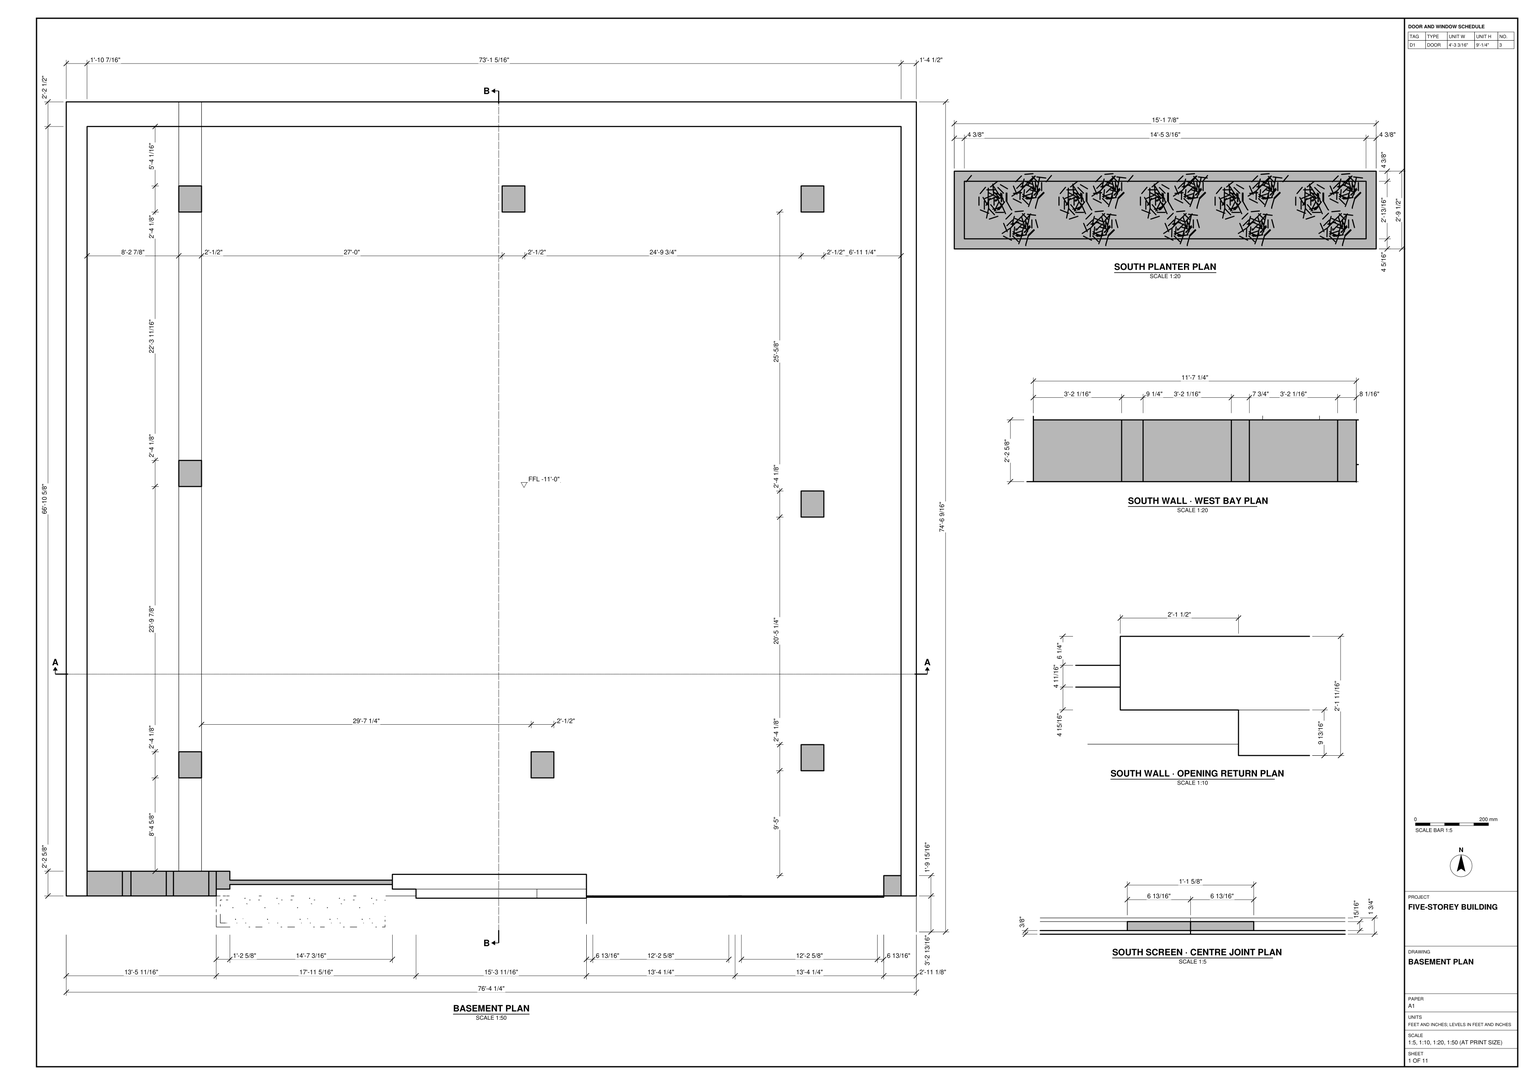
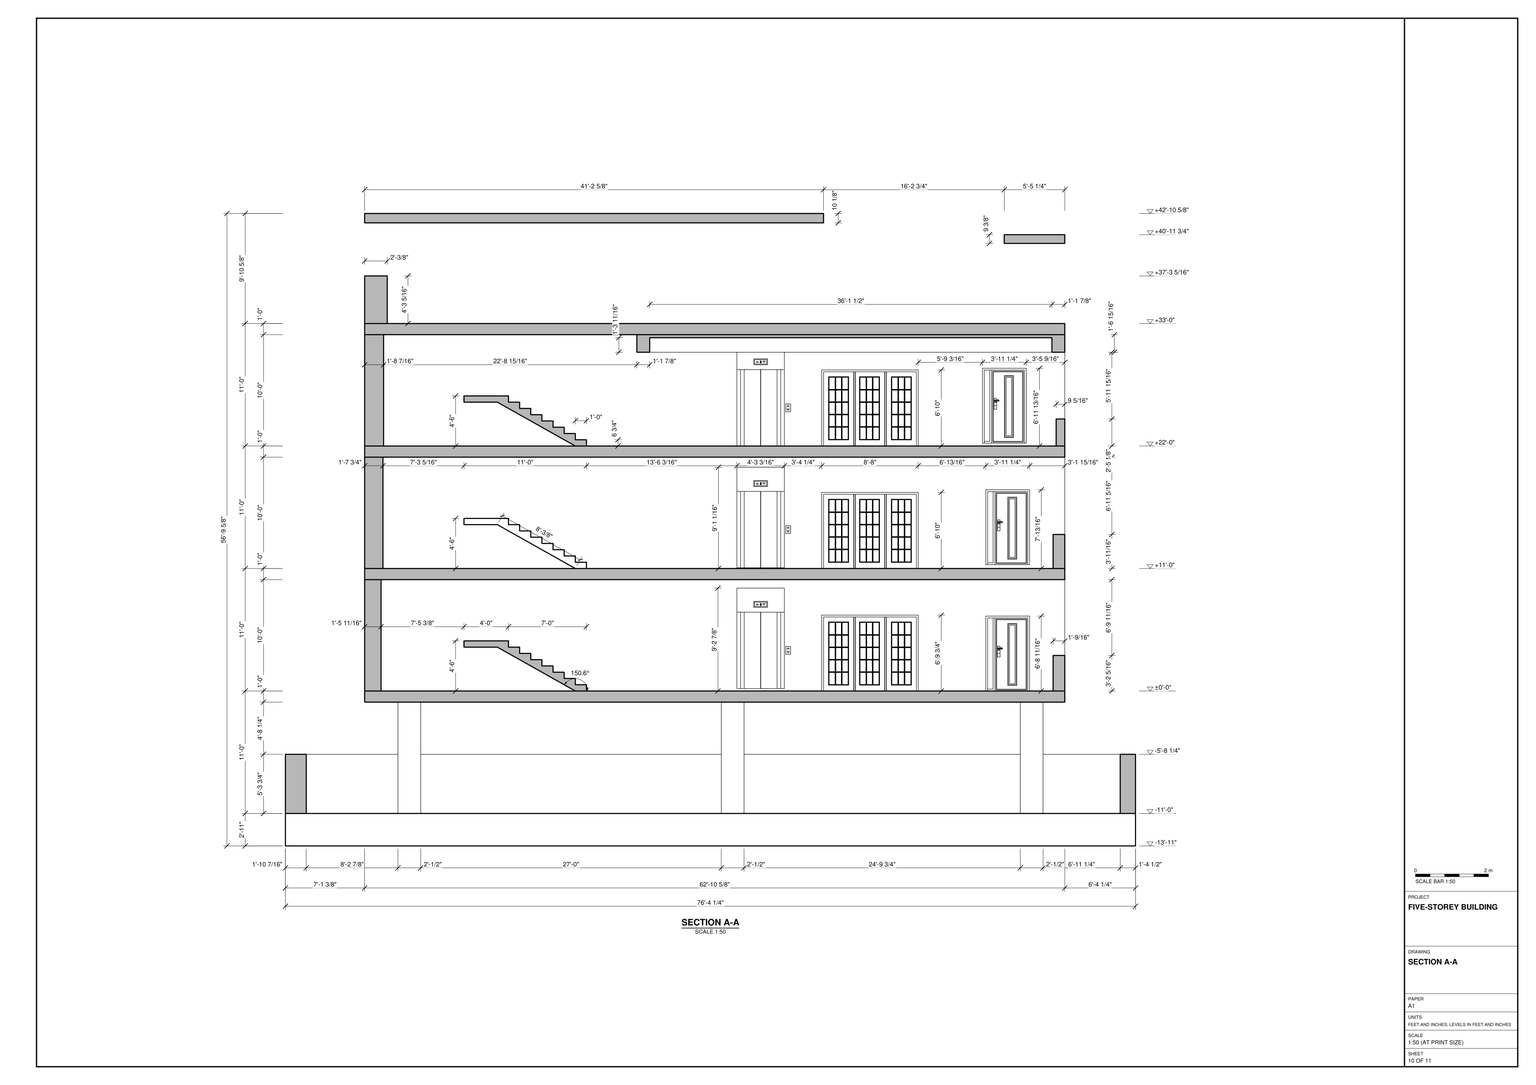
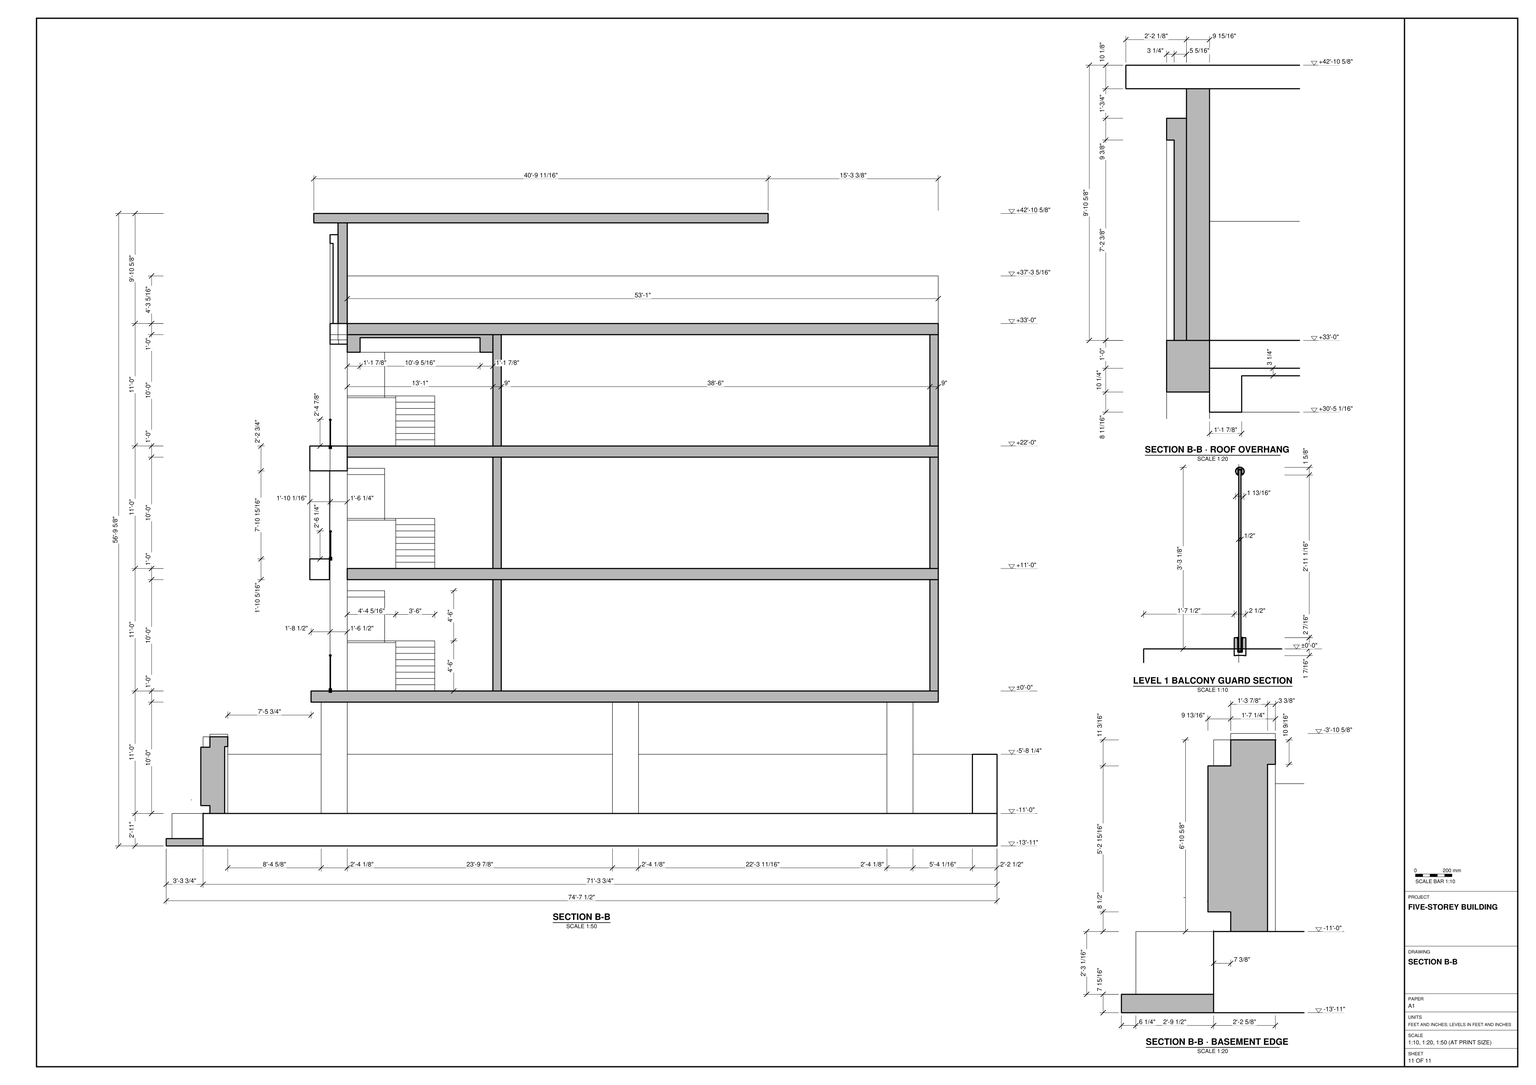
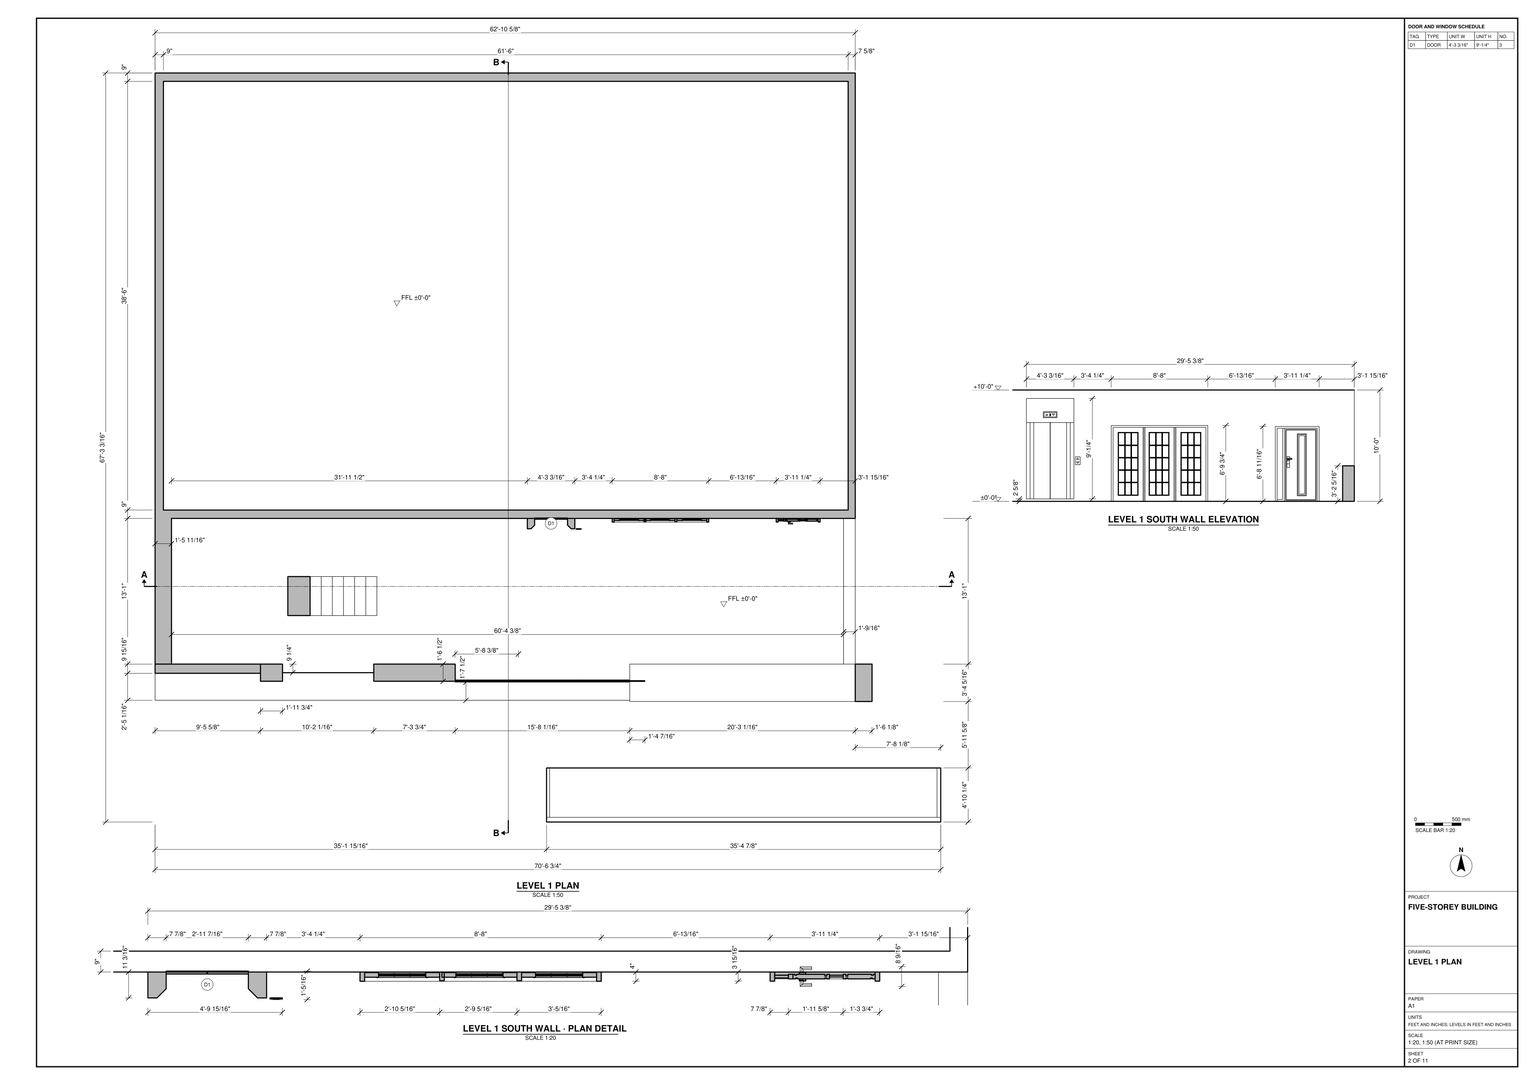
Build the five-storey building in SketchUp using task_files/diagram_01.pdf. Work in feet and inches. The complete model shall measure 77'-8 3/16" along X, 74'-8 5/8" along Y and 56'-9 5/8" along Z. Set the basement at -11'-0", the ground floor at ±0'-0", the next two floors at +11'-0" and +22'-0", and the roof terrace at +33'-0".

Use the basement plan to place the slab, perimeter walls and columns. Follow the details for the stepped wall return, screen and planter along the south side. Build the upper floor slabs, exterior walls and partitions with the thicknesses shown in section. Align the stair flights, landings and lift entrances with the floor plans. Use section A-A to place the tall divided-light openings and adjacent single doors on the occupied floors. Model the projecting balconies with their glass guards, and distinguish the open part of the roof terrace from the raised, overhanging roof above it.

Keep shell elements such as walls, slabs and roofs separate as groups or components. Model any built-in joinery and main furniture shown as separate pieces, and use components for repeated parts. Decor and loose items, including plants, may be any suitable library components. Save one SketchUp model as output_files/five_storey_building_with_balconies_and_a_roof_terrace.skp.

# SketchUp Ruby script. Lengths in inches.
U = 1.inch
M = Sketchup.active_model
def pt(a) = Geom::Point3d.new(a.map { |v| v * U })
def face(e, loops, mat)
  f = e.add_face(loops[0].map { |a| pt(a) })
  loops[1..].each { |l| e.add_face(l.map { |a| pt(a) }).erase! }
  f.material = f.back_material = mat if mat
  f
end
# faces: each face lists its corners as indices into pts; further lists are holes
def faces(e, pts, list, mat = nil) = list.each { |f| face(e, (f[0].is_a?(Array) ? f : [f]).map { |l| l.map { |i| pts[i] } }, mat) }
# xy, xz, yz: faces in a plane at the given z, y or x. An outline is a flat list of corners, or four numbers for a rectangle; further outlines are holes
def ring(l) = l.size == 4 ? [[l[0], l[1]], [l[2], l[1]], [l[2], l[3]], [l[0], l[3]]] : l.each_slice(2).to_a
def flat(e, list, mat, &to3) = list.each { |f| face(e, (f[0].is_a?(Array) ? f : [f]).map { |l| ring(l).map { |u, v| to3.(u, v) } }, mat) }
def xy(e, z, list, mat = nil) = flat(e, list, mat) { |x, y| [x, y, z] }
def xz(e, y, list, mat = nil) = flat(e, list, mat) { |x, z| [x, y, z] }
def yz(e, x, list, mat = nil) = flat(e, list, mat) { |y, z| [x, y, z] }
def lines(e, pts, list) = list.each { |a, b| e.add_line(pt(pts[a]), pt(pts[b])) }
# prism: a flat outline (further loops are holes) pulled along v
def prism(e, loops, v, mat = nil)
  f = face(e, loops, mat); d = Geom::Vector3d.new(v.map { |x| x * U })
  f.pushpull(f.normal.samedirection?(d) ? d.length : -d.length)
end
def box(e, o, s, mat = nil) = prism(e, [[o, [o[0] + s[0], o[1], o[2]], [o[0] + s[0], o[1] + s[1], o[2]], [o[0], o[1] + s[1], o[2]]]], [0, 0, s[2]], mat)
def at(x, y, z, deg = 0) = Geom::Transformation.translation(pt([x, y, z])) * Geom::Transformation.rotation(ORIGIN, Z_AXIS, deg.degrees)
def axes(o, x, y, z) = Geom::Transformation.new([*x, 0, *y, 0, *z, 0, *pt(o).to_a, 1])
def part(name) = M.definitions.add(name)
# library, detail: a bought-in or finely detailed component or shape, given as its bounding box
def library(name, o, s) = part(name).tap { |d| box(d.entities, o, s) }
def detail(e, o, s) = box(e.add_group.entities, o, s)
def put(e, d, t, mat = nil) = e.add_instance(d, t).tap { |i| i.material = mat if mat }
def group(e, t, mat = nil) = e.add_group.tap { |g| g.transformation = t; g.material = mat if mat }.entities
root = M.entities
M.materials.add("[Color C01]").color = [255, 229, 204]
M.materials.add("[Color C08]").color = [61, 30, 0]
M.materials.add("[Color M06]").color = [86, 86, 86]
M.materials.add("[Granite Dark Gray]").color = [69, 68, 68]
M.materials.add("[Granite Light Gray]").color = [234, 233, 226]
M.materials.add("[Translucent Glass Blue]").color = [100, 149, 237]
M.materials["[Translucent Glass Blue]"].alpha = 0.5
M.materials.add("[Wood Bamboo]").color = [177, 105, 43]
M.materials.add("[Wood Cherry Original]").color = [152, 86, 42]
M.materials.add("hymenocallis littoralis").color = [156, 172, 146]
c1 = library("staircase",[119.25,98.03,0],[96,132,108])
c2 = library("ประตู",[99.61,0,0],[47.24,8.5625,80.71])
c3 = library("Wagner Glass Railing",[9.08,102.375,1.53],[2.51,145.5,42.05])
c4 = library("Untitled",[1.05,171.5,-132],[104,4,82])
c5 = library("lift",[-933.37,365.14,432],[57.92,12.32,108.27])
c6 = library("Porton casa",[225.62,-50.57,0],[86.62,1.75,86.61])
c7 = part("Group\#856")
xy(c7.entities,7.38,[[0,0,5.5,15.91]],"hymenocallis littoralis")
p = [[5.5,28.78,0],[5.5,26.79,3.44],[0,26.79,3.44],[0,28.78,0],[0,23.75,6],[5.5,23.75,6],
  [0,15.91,7.38],[5.5,15.91,7.38]]
faces(c7.entities,p,[[0,1,2,3],[4,2,1,5],[6,4,5,7]],"hymenocallis littoralis")
c8 = part("Group\#854")
xy(c8.entities,7.38,[[0,0,5.5,15.91],[0,15.91,5.5,23.87]],"hymenocallis littoralis")
p = [[5.5,31.07,4.3],[5.5,27.74,6.47],[0,27.74,6.47],[0,31.07,4.3],[0,23.87,7.38],[5.5,23.87,7.38]]
faces(c8.entities,p,[[0,1,2,3],[4,2,1,5]],"hymenocallis littoralis")
c9 = part("Group\#857")
xy(c9.entities,7.38,[[0,0,5.6,15.91]],"hymenocallis littoralis")
p = [[5.6,28.78,0],[5.6,26.79,3.44],[0,26.79,3.44],[0,28.78,0],[0,23.75,6],[5.6,23.75,6],
  [0,15.91,7.38],[5.6,15.91,7.38]]
faces(c9.entities,p,[[0,1,2,3],[4,2,1,5],[6,4,5,7]],"hymenocallis littoralis")
c10 = part("Group\#855")
put(c10.entities,c8,axes([6.09,8.57,-0.52],[0.446,0.85617,0.26089],[-0.18444,-0.19731,0.96283],[0.87582,-0.47754,0.0699]))
put(c10.entities,c8,axes([6.29,7.28,-1.71],[0.37058,0.92707,-0.05667],[-0.32382,0.19004,0.99128],[0.87712,-0.32925,0.34964]))
put(c10.entities,c8,axes([11.04,16.14,-0.7],[1,0,0],[0,0.16628,1.02662],[0,-1.18456,0.19186]))
c11 = part("Group\#860")
put(c11.entities,c7,axes([24.57,32.05,-1.76],[0.9552,-0.22102,-0.19681],[0.4036,0.95545,0.88585],[-0.00568,-0.67859,0.7345]))
put(c11.entities,c7,axes([23.95,29.24,-2.4],[0,1,0],[-0.76041,0,0.64945],[0.64945,0,0.76041]))
put(c11.entities,c7,axes([24.22,24.72,-0.48],[-0.70711,0.70711,0],[-0.32757,-0.32757,0.80237],[0.61237,0.61237,0.5]))
put(c11.entities,c8,axes([20.66,37.22,-0.63],[1.12361,0.03262,0.39091],[-0.43499,0.29739,0.78777],[0.09852,-1.27434,0.37535]))
put(c11.entities,c7,axes([28.75,24.45,-2.4],[-1,0,0],[0,-0.76041,0.64945],[0,0.64945,0.76041]))
put(c11.entities,c9,axes([30.4,30.98,-3.7],[0.65676,-0.72002,0.22414],[0.55667,0.66341,0.5],[-0.50871,-0.20361,0.83652]))
put(c11.entities,c9,axes([32.41,29.61,-3.7],[0.04029,-0.97372,0.22414],[0.85287,0.15038,0.5],[-0.52057,0.17102,0.83652]))
put(c11.entities,c7,axes([31.89,25.85,-1.76],[-0.92056,0.33739,-0.19681],[-0.5186,-0.89824,0.88585],[0.08952,0.67268,0.7345]))
put(c11.entities,c7,axes([25.55,34.78,-0.48],[0.86603,0.5,0],[-0.25,0.43301,0.86603],[0.43301,-0.75,0.5]))
put(c11.entities,c9,axes([20.4,16.9375,-8.07],[-0.70711,0.70711,0],[-0.35754,-0.35754,0.65422],[1.3987,1.3987,1.52882]))
put(c11.entities,c7,axes([32.86,34.14,-0.48],[0.76604,-0.64279,0],[0.32139,0.38302,0.86603],[-0.55667,-0.66341,0.5]))
put(c11.entities,c7,axes([27.15,34.7,-0.1],[0.82472,-0.17528,-0.53769],[0.53769,0.53769,0.64945],[0.17528,-0.82472,0.53769]))
put(c11.entities,c7,axes([33.58,28.77,-2.4],[0,-1,0],[0.76041,0,0.64945],[-0.64945,0,0.76041]))
put(c11.entities,c7,axes([26.43,23.87,-2.81],[-0.75126,0.04415,0.65853],[0.53769,-0.53769,0.64945],[0.38276,0.84199,0.3802]))
put(c11.entities,c7,axes([28.78,23.98,-2.4],[-1,0,0],[0,-0.76041,0.64945],[0,0.64945,0.76041]))
put(c11.entities,c7,axes([25.39,25.38,-2.4],[-0.70711,0.70711,0],[-0.53769,-0.53769,0.64945],[0.45923,0.45923,0.76041]))
put(c11.entities,c7,axes([27.32,21.63,-0.1],[-0.45923,0.70711,-0.53769],[-0.76041,0,0.64945],[0.45923,0.70711,0.53769]))
put(c11.entities,c7,axes([25.17,27.625,-1.76],[0.56416,0.80187,-0.19681],[-0.66673,0.66673,0.80532],[0.62659,-0.26057,0.7345]))
put(c11.entities,c9,axes([27.59,27.04,-3.96],[-0.8993,-0.06127,0.43301],[0.2962,-0.8138,0.5],[0.32175,0.57791,0.75]))
put(c11.entities,c9,axes([26.98,24.5,-3.18],[-0.5,0.86603,0],[-0.75,-0.43301,0.5],[0.43301,0.25,0.86603]))
put(c11.entities,c9,axes([24.55,27.74,-3.7],[0.29517,0.92878,0.22414],[-0.85287,0.15038,0.5],[0.43068,-0.33875,0.83652]))
put(c11.entities,c9,axes([24.26,29.8,-3.18],[0.76604,0.64279,0],[-0.47317,0.5639,0.425],[0.32139,-0.38302,0.86603]))
put(c11.entities,c9,axes([25.98,32.46,-3.18],[1,0,0],[0,0.86603,0.5],[0,-0.5,0.86603]))
put(c11.entities,c7,axes([28.78,33.57,-2.4],[1,0,0],[0,0.76041,0.64945],[0,-0.64945,0.76041]))
put(c11.entities,c10,at(14.99,21.38,2.5))
put(c11.entities,c8,axes([34.63,26.34,-1.46],[-0.70089,-0.70877,0.07994],[0.4756,-0.38088,0.79293],[-0.53156,0.59378,0.60405]))
put(c11.entities,c8,axes([28.14,16.92,1.8125],[-1.19719,0.6912,0],[-0.09607,-0.16641,0.94244],[0.68444,1.18549,0.17613]))
put(c11.entities,c8,axes([31.5625,35.84,0.97],[0.66765,-1.1564,0.35779],[0.04445,0.30732,0.91033],[-1.20828,-0.64496,0.17012]))
put(c11.entities,c8,axes([38.94,22.51,0.89],[-0.97932,-0.67164,-0.05202],[0.27787,-0.41401,0.90999],[-0.85985,0.93577,0.32097]))
put(c11.entities,c8,axes([38.44,21.09,1.98],[-1.02864,-0.54856,0.2395],[0.33481,0.06999,0.88388],[-0.77261,1.08328,0.06417]))
put(c11.entities,c9,axes([35.02,30.51,-1.3],[-0.17365,-0.98481,0],[0.60224,-0.10619,0.79122],[-0.7792,0.13739,0.61153]))
put(c11.entities,c9,axes([29.41,22.33,-1.3],[-0.93969,0.34202,0],[-0.20915,-0.57465,0.79122],[0.27061,0.74351,0.61153]))
put(c11.entities,c8,axes([19.64,36,-1.62],[1.18194,0.09546,0.08234],[-0.14377,0.68823,0.76313],[0.21457,-1.1326,0.62386]))
put(c11.entities,c9,axes([24.25,24.14,-1.3],[-0.34202,0.93969,0],[-0.57465,-0.20915,0.79122],[0.74351,0.27061,0.61153]))
put(c11.entities,c9,axes([25.98,34.61,-1.3],[1,0,0],[0,0.61153,0.79122],[0,-0.79122,0.61153]))
put(c11.entities,c9,axes([31.16,34.41,-1.64],[0.56518,-0.80224,-0.19234],[0.73413,0.34233,0.72935],[-0.47639,-0.50772,0.71782]))
put(c11.entities,c9,axes([40.52,26.84,-5.82],[-0.42262,-0.90631,0],[0.48019,-0.22391,0.68552],[-1.43418,0.66877,1.22305]))
put(c11.entities,c7,axes([29.86,38.42,-1.01],[0.89064,-0.37013,0.26413],[-0.03924,0.63286,1.01918],[-0.45353,-0.76487,0.45748]))
put(c11.entities,c7,axes([29.34,22.4,-0.48],[-0.99619,-0.08716,0],[0.04358,-0.4981,0.86603],[-0.07548,0.86273,0.5]))
c12 = part("Group\#858")
xz(c12.entities,10.07,[[9.07,0,10.07,31.01],[0,31.01,0,45.12,20.13,45.12,20.13,31.01,10.07,31.01,10.07,32.58,9.07,32.58,9.07,31.01]],"hymenocallis littoralis")
yz(c12.entities,10.07,[[0,31.01,20.13,45.12]],"hymenocallis littoralis")
p = [[9.57,9.2,0],[10.07,10.07,0],[10.07,10.07,31.01],[10.07,10.07,32.58],[9.57,9.2,32.58]]
faces(c12.entities,p,[[0,1,2,3,4]],"hymenocallis littoralis")
c13 = part("cây lá nắng")
put(c13.entities,c11,axes([49.26,-2.75,0],[0.63109,0.63109,0],[-0.63109,0.63109,0],[0,0,0.935]))
g1 = group(c13.entities,at(26.6,-8.68,0))
put(g1,c7,axes([-4.72,35.73,-1.65],[0.74231,0.46334,-0.18402],[-0.34827,0.85768,0.82827],[0.42467,-0.43184,0.68675]))
put(g1,c7,axes([-3.34,33.57,-2.24],[-0.63109,0.63109,0],[-0.47989,-0.47989,0.60723],[0.40986,0.40986,0.71098]))
put(g1,c7,axes([-0.3125,30.89,-0.45],[-0.8925,0,0],[0,-0.41345,0.75022],[0,0.77293,0.4675]))
put(g1,c8,axes([-10.79,39.66,-0.59],[0.68852,0.72969,0.3655],[-0.4622,-0.08684,0.73657],[0.86641,-0.74205,0.35095]))
put(g1,c7,axes([2.71,33.57,-2.24],[-0.63109,-0.63109,0],[0.47989,-0.47989,0.60723],[-0.40986,0.40986,0.71098]))
put(g1,c9,axes([-0.37,38.74,-3.46],[0.86887,-0.03992,0.20957],[-0.06737,0.76999,0.4675],[-0.19255,-0.44954,0.78214]))
put(g1,c9,axes([1.76,39.14,-3.46],[0.63993,-0.58908,0.20957],[0.44333,0.63315,0.4675],[-0.43646,-0.2206,0.78214]))
put(g1,c7,axes([3.81,36.4375,-1.65],[-0.79389,-0.36803,-0.18402],[0.23959,-0.89415,0.82827],[-0.36803,0.48102,0.68675]))
put(g1,c7,axes([-5.83,38.07,-0.45],[0.231,0.86209,0],[-0.43104,0.1155,0.80973],[0.74659,-0.20005,0.4675]))
put(g1,c9,axes([2.18,23.5625,-7.55],[-0.8925,0,0],[0,-0.45128,0.6117],[0,1.76542,1.42944]))
put(g1,c7,axes([-0.8125,42.28,-0.45],[0.8891,0.07779,0],[-0.03889,0.44455,0.80973],[0.06737,-0.76999,0.4675]))
put(g1,c7,axes([-4.76,39.03,-0.09],[0.63109,0.40986,-0.50274],[0,0.67866,0.60723],[0.63109,-0.40986,0.50274]))
put(g1,c7,axes([3.03,39.35,-2.24],[0.63109,-0.63109,0],[0.47989,0.47989,0.60723],[-0.40986,-0.40986,0.71098]))
put(g1,c7,axes([1.61,31.74,-2.625],[-0.50198,-0.44625,0.61573],[0.67866,0,0.60723],[-0.28982,0.77293,0.35549]))
put(g1,c7,axes([3.03,33.3,-2.24],[-0.63109,-0.63109,0],[0.47989,-0.47989,0.60723],[-0.40986,0.40986,0.71098]))
put(g1,c7,axes([0.01,32.04,-2.24],[-0.8925,0,0],[0,-0.67866,0.60723],[0,0.57963,0.71098]))
put(g1,c7,axes([3.59,30.89,-0.09],[-0.73607,0.15643,-0.50274],[-0.47989,-0.47989,0.60723],[-0.15643,0.73607,0.50274]))
put(g1,c7,axes([-1.55,33.32,-1.65],[-0.15002,0.86209,-0.18402],[-0.84154,0,0.75297],[0.55988,0.231,0.68675]))
put(g1,c9,axes([0.35,34.48,-3.71],[-0.52887,-0.60621,0.40487],[0.70051,-0.32665,0.4675],[-0.16166,0.56777,0.70125]))
put(g1,c9,axes([2.61,39.13,-1.74],[-0.86209,0.231,0],[-0.23031,-0.85954,0.15531],[0.03162,0.11799,0.91645]))
put(g1,c9,axes([-2.02,33,-3.46],[-0.39986,0.77243,0.20957],[-0.63315,-0.44333,0.4675],[0.48558,0.05802,0.78214]))
put(g1,c9,axes([-3.49,34.12,-2.97],[0.07779,0.8891,0],[-0.65449,0.05726,0.39737],[0.44455,-0.03889,0.80973]))
put(g1,c9,axes([-4.09,36.88,-2.97],[0.63109,0.63109,0],[-0.54654,0.54654,0.4675],[0.31555,-0.31555,0.80973]))
put(g1,c7,axes([-3.02,39.35,-2.24],[0.63109,0.63109,0],[-0.47989,0.47989,0.60723],[0.40986,-0.40986,0.71098]))
put(g1,c10,axes([-4.03,22.95,2.33],[0.63109,0.63109,0],[-0.63109,0.63109,0],[0,0,0.935]))
put(g1,c8,axes([5.24,38.48,-1.37],[0.00497,-0.88963,0.07474],[0.54052,0.05978,0.74139],[-0.71019,0.03927,0.56479]))
put(g1,c8,axes([7.08,28.4375,1.7],[-1.19175,-0.31933,0],[0.04439,-0.16565,0.88118],[-0.31621,1.1801,0.16468]))
put(g1,c8,axes([-2.7,42.54,0.91],[1.15114,-0.30845,0.33454],[-0.1659,0.22199,0.85115],[-0.3555,-1.16957,0.15907]))
put(g1,c8,axes([10.37,38.78,0.83],[-0.19417,-1.04191,-0.04864],[0.43664,-0.08592,0.85084],[-1.1332,0.04791,0.30011]))
put(g1,c8,axes([10.95,37.5625,1.85],[-0.30298,-0.99536,0.22393],[0.16713,0.25547,0.82643],[-1.17124,0.19607,0.06]))
put(g1,c9,axes([2.84,41.36,-1.22],[0.51192,-0.73109,0],[0.44708,0.31305,0.73979],[-0.57846,-0.40504,0.57178]))
put(g1,c9,axes([4.47,32.65,-1.22],[-0.80888,-0.37719,0],[0.23066,-0.49465,0.73979],[-0.29844,0.64,0.57178]))
put(g1,c8,axes([-10.32,35.12,-1.51],[0.68567,0.80616,0.07699],[-0.52507,0.3436,0.71352],[0.85019,-0.57936,0.58331]))
put(g1,c9,axes([0.07,30.54,-1.22],[-0.80888,0.37719,0],[-0.23066,-0.49465,0.73979],[0.29844,0.64,0.57178]))
put(g1,c9,axes([-5.45,38.24,-1.22],[0.63109,0.63109,0],[-0.38593,0.38593,0.73979],[0.49934,-0.49934,0.57178]))
put(g1,c9,axes([-2.05,41.38,-1.53],[0.86296,-0.14961,-0.17984],[0.24726,0.67935,0.68194],[0.01977,-0.62107,0.67116]))
put(g1,c9,axes([8.63,42.51,-5.4375],[0.30525,-0.83868,0],[0.44435,0.16173,0.64096],[-1.32716,-0.48305,1.14356]))
put(g1,c7,axes([-5.4,43.09,-0.94],[0.79566,0.32849,0.24696],[-0.42416,0.37462,0.95293],[0.19648,-0.76892,0.42774]))
put(g1,c7,axes([4.38,32.65,-0.45],[-0.57369,-0.68369,0],[0.34185,-0.28684,0.80973],[-0.5921,0.49683,0.4675]))
put(g1,c9,axes([-2,33.84,-0.15],[-0.24601,0.85793,0],[-0.85539,-0.24528,0.15531],[0.11742,0.03367,0.91645]))
put(g1,c9,axes([0.17,30.83,-4.47],[-0.24601,0.85793,0],[-0.85539,-0.24528,0.15531],[0.11742,0.03367,0.91645]))
put(g1,c9,axes([-1.97,32.18,-4.47],[0.58524,0.67383,0],[-0.67184,0.58351,0.15531],[0.09222,-0.0801,0.91645]))
put(g1,c9,axes([-2,34.71,-4.47],[0.88392,-0.12346,0],[0.12309,0.88131,0.15531],[-0.0169,-0.12098,0.91645]))
put(g1,c9,axes([0.11,36.12,-4.47],[0.37822,-0.8084,0],[0.80601,0.37711,0.15531],[-0.11064,-0.05177,0.91645]))
put(c13.entities,c12,axes([29.71,14.29,6.94],[0.425,0.73612,0],[-0.6771,0.39092,-0.33349],[-0.26859,0.15507,0.72712]))
put(c13.entities,c12,axes([42.0625,26.12,6.94],[0.85,0,0],[0,0.78185,-0.33349],[0,0.33349,0.78185]))
put(c13.entities,c11,axes([7.3125,23.0625,0],[0.8925,0,0],[0,0.8925,0],[0,0,0.935]))
put(c13.entities,c12,axes([24.4375,40.23,2.05],[0.85,0,0],[0,0.85,0],[0,0,0.85]))
c14 = part("Planting 101")
put(c14.entities,c13,axes([21.34,32.96,-4.59],[0,-0.71,0],[-0.71,0,0],[0,0,0.71]))
c15 = part("Group\#17")
box(c15.entities,[0,0,0],[24.5,28.125,120])
c16 = part("Group\#18")
box(c16.entities,[0,0,0],[38.0625,26.625,82.625])
box(root,[60.51,40.875,-132],[55.06,26.625,67.3],"[Color M06]")
xy(root,-167,[[0.74,1.125,560.68,40.875],[560.68,2.0625,916.25,40.875]])
xy(root,-159.0625,[[0.74,1.125,560.68,1.125,560.68,40.875,343.6,40.875,343.6,7.375,161.7,7.375,161.7,40.875,0.74,40.875],[161.7,7.375,343.6,40.875]])
xy(root,-145.1875,[[166.04,11.72,339.25,36.53]])
xy(root,-132,[[[161.7,7.375,343.6,40.875],[166.04,11.72,339.25,36.53]]])
xy(root,-132,[[0,40.875,0,896.625,916.25,896.625,916.25,40.875,899.77,40.875,899.77,870.1,22.45,870.1,22.45,40.875],[153.64,40.875,161.7,67.5],[881.15,40.875,899.77,62.8],[161.7,48.25,161.7,67.5,176.32,67.5,176.32,57.875,351.51,57.875,351.51,53.18,176.32,53.18,176.32,48.25],[351.51,48.25,560.68,64.125]],"[Color M06]")
xy(root,-123.52,[[376.99,38.4375,507.32,48.25],[507.32,38.4375,560.68,48.25]],"[Color M06]")
xy(root,-69.14,[[153.64,40.875,161.7,67.5]],"[Color M06]")
xy(root,-68.25,[[0,40.875,22.45,40.875,22.45,870.1,899.77,870.1,899.77,40.875,916.25,40.875,916.25,896.625,0,896.625]],"[Color M06]")
xy(root,-60.59,[[376.99,38.4375,507.32,48.25],[507.32,38.4375,560.68,48.25]],"[Color M06]")
xy(root,-59.95,[[176.32,48.25,351.51,53.18],[176.32,57.875,176.32,67.5,507.32,67.5,507.32,64.125,351.51,64.125,351.51,57.875]],"[Color M06]")
xy(root,-49.375,[[161.7,48.25,351.51,67.5],[378.18,48.25,507.32,67.5]],"[Color M06]")
xy(root,-46.625,[[351.51,48.25,378.18,67.5]],"[Color M06]")
xy(root,-12,[[199.01,177.75,408.87,196.25],[85.4,186.3125,199.01,196.25]],"[Color M06]")
xy(root,-3.21,[[222.78,177.75,321.09,187],[222.78,187,321.09,196.25]],"[Color M06]")
xy(root,0,[[827.44,196.25,840.03,353.25]])
xy(root,0,[[596.96,170,840.03,196.25],[85.4,196.25,103.1,353.25],[[85.4,353.25,840.03,833.25],[94.4,362.25,832.4,824.25]],[94.4,362.25,832.4,824.25]],"[Color M06]")
xy(root,10,[[596.96,155.9375,596.96,170,840.03,170,840.03,196.25,858.15,196.25,858.15,155.9375],[596.96,170,840.03,196.25]],"[Color M06]")
xy(root,27.75,[[881.15,40.875,899.77,62.8],[507.32,48.25,560.68,64.125],[507.32,64.125,560.68,84.3125]],"[Color M06]")
xy(root,27.75,[[507.32,26.0625,560.68,48.25],[560.68,26.0625,560.68,84.3125,932.18,84.3125,932.18,26.0625,899.77,26.0625,899.77,62.8,881.15,62.8,881.15,26.0625],[881.15,26.0625,899.77,40.875]],"[Wood Cherry Original]")
xy(root,35.6875,[[507.32,26.0625,932.18,31.0625],[507.32,31.0625,510.64,84.3125],[510.64,31.0625,928.18,84.3125],[928.18,31.0625,932.18,84.3125]],"[Color M06]")
xy(root,38.3125,[[827.44,196.25,840.03,353.25]])
xy(root,39.18,[[596.96,155.9375,840.03,196.25]],"[Color M06]")
xy(root,43.625,[[507.32,26.0625,932.18,31.0625],[507.32,31.0625,510.64,84.3125],[510.64,31.0625,928.18,84.3125],[928.18,31.0625,932.18,84.3125]],"[Color M06]")
xy(root,50.8125,[[507.32,26.0625,932.18,84.3125]],"[Color M06]")
xy(root,79.68,[[85.4,186.3125,199.01,190.3125]],"[Color M06]")
xy(root,84.31,[[85.4,186.3125,199.01,190.3125]],"[Color M06]")
xy(root,105.72,[[222.78,177.75,321.09,187],[222.78,187,321.09,196.25]],"[Color M06]")
xy(root,120,[[348.63,155.9375,840.03,177],[85.4,196.25,103.1,353.25],[[85.4,353.25,840.03,833.25],[94.4,362.25,832.4,824.25]]],"[Color M06]")
xy(root,132,[[827.4375,196.25,840.03,353.25]])
xy(root,132,[[85.4,196.25,105.13,353.25],[[85.4,353.25,840.03,833.25],[94.4,362.25,832.4,824.25]],[94.4,362.25,832.4,824.25]],"[Color M06]")
xy(root,136.1,[[222.78,177.75,321.09,187],[222.78,187,321.09,196.25]],"[Color M06]")
xy(root,142.33,[[409.26,155.9375,840.03,177]],"[Color M06]")
xy(root,168.6875,[[827.4375,196.25,840.03,353.25]])
xy(root,177.92,[[85.4,186.3125,199.01,190.3125]],"[Color M06]")
xy(root,181.03,[[85.4,186.3125,199.01,190.3125]],"[Color M06]")
xy(root,237.25,[[409.26,155.9375,409.26,177,348.63,177,348.63,196.25,840.03,196.25,840.03,155.9375]],"[Color M06]")
xy(root,245.04,[[222.78,177.75,321.09,187],[222.78,187,321.09,196.25]],"[Color M06]")
xy(root,252,[[85.4,196.25,105.13,353.25],[[85.4,353.25,840.03,833.25],[94.4,362.25,832.4,824.25]]],"[Color M06]")
xy(root,264,[[830.7,196.25,840.03,353.25]])
xy(root,264,[[348.63,155.9375,615.23,196.25],[615.23,155.9375,840.03,161.4375],[615.23,161.4375,840.03,196.25],[85.4,196.25,105.82,353.25],[[85.4,353.25,840.03,833.25],[94.4,362.25,832.4,824.25]],
  [94.4,362.25,832.4,824.25]],"[Color M06]")
xy(root,269.47,[[222.78,177.75,321.09,187],[222.78,187,321.09,196.25]],"[Color M06]")
xy(root,271.39,[[85.4,186.3125,199.01,190.3125]],"[Color M06]")
xy(root,273.55,[[85.4,186.3125,199.01,190.3125]],"[Color M06]")
xy(root,280.8125,[[615.23,155.9375,840.03,161.4375],[615.23,161.4375,840.03,196.25]],"[Color M06]")
xy(root,293.125,[[830.7,196.25,840.03,353.25]])
xy(root,304.6875,[[615.23,155.9375,858.15,196.25]],"[Color M06]")
xy(root,352.51,[[85.4,186.3125,199.01,190.3125]],"[Color M06]")
xy(root,354.87,[[85.4,186.3125,199.01,190.3125]],"[Color M06]")
xy(root,365.0625,[[[378.79,196.25,840.03,353.25],[392.65,210.11,826.17,339.39]]],"[Wood Cherry Original]")
xy(root,373.75,[[408.87,177.75,840.03,196.25]],"[Color C08]")
xy(root,378.41,[[222.78,177.75,321.09,187],[222.78,187,321.09,196.25]],"[Color M06]")
xy(root,380.75,[[392.65,210.11,826.17,339.39]],"[Wood Cherry Original]")
xy(root,384,[[85.4,196.25,105.82,353.25],[378.79,196.25,840.03,353.25],[[85.4,353.25,840.03,833.25],[94.4,362.25,832.4,824.25]]],"[Color M06]")
xy(root,396,[[199.01,177.75,337.61,186.3125],[337.61,177.75,350.68,177.75,350.68,181,840.03,181,840.03,186.3125,337.61,186.3125],[350.68,177.75,384.01,181],[384.01,177.75,840.03,181],[199.01,186.3125,580.01,196.25],
  [580.01,186.3125,840.03,196.25],[85.4,196.25,109.75,833.25]],"[Color M06]")
xy(root,406.82,[[580.01,181,840.03,186.3125]],"[Wood Cherry Original]")
xy(root,447.05,[[85.4,186.3125,337.61,189.25]],"[Color M06]")
xy(root,447.3125,[[85.4,196.25,109.75,833.25]],"[Color M06]")
xy(root,449.0625,[[85.4,186.3125,337.61,189.25]],"[Color M06]")
xy(root,482.36,[[350.68,177.75,350.68,181,580.01,181,840.03,177.75],[840.03,177.75,580.01,181,580.01,256.0625,774.75,256.0625,774.75,833.25,840.03,833.25]],"[Wood Cherry Original]")
xy(root,491.75,[[337.61,177.75,840.03,177.75,580.01,181,580.01,186.3125,337.61,186.3125],[840.03,177.75,840.03,833.25,774.75,833.25,774.75,256.0625,580.01,256.0625,580.01,181]],"[Wood Cherry Original]")
xy(root,504.5,[[85.4,186.3125,580.01,196.25],[85.4,196.25,580.01,649.875]],"[Color M06]")
xy(root,504.5,[[85.4,160.1875,580.01,186.3125]],"[Wood Cherry Original]")
xy(root,514.625,[[85.4,160.1875,580.01,649.875]],"[Color M06]")
xz(root,1.125,[[0.74,-167,560.68,-159.0625]])
xz(root,7.375,[[161.7,-159.0625,343.6,-132]])
xz(root,11.72,[[166.04,-145.1875,339.25,-132]])
xz(root,26.0625,[[507.32,27.75,932.18,35.6875],[507.32,43.625,932.18,50.8125]],"[Color M06]")
xz(root,31.0625,[[510.64,35.6875,928.18,43.625]],"[Color M06]")
xz(root,36.53,[[166.04,-145.1875,339.25,-132]])
xz(root,38.4375,[[376.99,-120.68,406.93,-62.75]],"[Color M06]")
xz(root,38.4375,[[376.99,-123.52,560.68,-123.52,560.68,-60.59,376.99,-60.59,376.99,-62.75,406.93,-62.75,406.93,-120.68,376.99,-120.68]],"[Granite Dark Gray]")
xz(root,40.875,[[0.74,-167,560.68,-159.0625],[560.68,-167,916.25,-132],[161.7,-159.0625,343.6,-132]])
xz(root,40.875,[[0,-132,22.45,-68.25],[153.64,-132,161.7,-69.14],[881.15,-132,899.77,27.75],[899.77,-132,916.25,-68.25]],"[Color M06]")
xz(root,48.25,[[161.7,-132,176.32,-132,176.32,-59.95,351.51,-59.95,351.51,-49.375,161.7,-49.375],[351.51,-132,507.32,-132,507.32,-123.52,376.99,-123.52,376.99,-60.59,507.32,-60.59,507.32,-49.375,378.18,-49.375,378.18,-46.625,351.51,-46.625],[507.32,-132,560.68,-123.52],[507.32,-60.59,560.68,27.75]],"[Color M06]")
xz(root,53.18,[[176.32,-132,351.51,-59.95]],"[Wood Bamboo]")
xz(root,57.875,[[176.32,-132,351.51,-59.95]],"[Color M06]")
xz(root,62.8,[[881.15,-132,899.77,27.75]],"[Color M06]")
xz(root,64.125,[[351.51,-132,351.51,-59.95,507.32,-59.95,507.32,27.75,560.68,27.75,560.68,-132],[351.51,-59.95,507.32,-59.9375]],"[Color M06]")
xz(root,67.5,[[153.64,-132,161.7,-69.14],[161.7,-132,161.7,-49.375,351.51,-49.375,351.51,-46.625,378.18,-46.625,378.18,-49.375,507.32,-49.375,507.32,-59.95,176.32,-59.95,176.32,-132]],"[Color M06]")
xz(root,84.3125,[[507.32,27.75,932.18,35.6875],[510.64,35.6875,928.18,43.625],[507.32,43.625,932.18,50.8125]],"[Color M06]")
xz(root,155.9375,[[348.63,120,840.03,120,840.03,142.33,409.26,142.33,409.26,237.25,840.03,237.25,840.03,264,348.63,264]],"[Color C01]")
xz(root,155.9375,[[596.96,10,858.15,10,858.15,304.6875,615.23,304.6875,615.23,280.8125,840.03,280.8125,840.03,39.18,596.96,39.18]],"[Color M06]")
xz(root,160.1875,[[85.4,504.5,580.01,514.625]],"[Color M06]")
xz(root,161.4375,[[615.23,264,840.03,280.8125]],"[Color M06]")
xz(root,170,[[596.96,0,840.03,10]],"[Color M06]")
xz(root,177,[[348.63,120,348.63,237.25,409.26,237.25,409.26,142.33,840.03,142.33,840.03,120]],"[Color M06]")
xz(root,177.75,[[[199.01,-12,408.87,-12,408.87,373.75,840.03,373.75,840.03,396,199.01,396],[222.78,-3.21,321.09,105.72],[222.78,136.1,321.09,245.04],[222.78,269.47,321.09,378.41]]],"[Color C08]")
xz(root,177.75,[[337.61,396,350.68,396,350.68,482.36,840.03,482.36,840.03,491.75,337.61,491.75]],"[Wood Cherry Original]")
xz(root,181,[[350.68,396,840.03,396,840.03,406.82,580.01,406.82,580.01,482.36,350.68,482.36]],"[Wood Cherry Original]")
xz(root,186.3125,[[337.61,396,580.01,491.75]],"[Color M06]")
xz(root,186.3125,[[85.4,-12,199.01,79.68],[85.4,84.31,199.01,177.92],[85.4,181.03,199.01,271.39],[85.4,273.55,199.01,352.51],[85.4,354.87,199.01,354.87,199.01,396,337.61,396,337.61,447.05,85.4,447.05],
  [85.4,449.0625,337.61,449.0625,337.61,491.75,580.01,491.75,580.01,504.5,85.4,504.5]],"[Granite Light Gray]")
xz(root,186.3125,[[580.01,396,840.03,406.82]],"[Wood Cherry Original]")
xz(root,187,[[222.78,-3.21,321.09,105.72],[222.78,136.1,321.09,245.04],[222.78,269.47,321.09,378.41]],"[Translucent Glass Blue]")
xz(root,189.25,[[85.4,447.05,337.61,449.0625]],"[Color M06]")
xz(root,190.3125,[[85.4,79.68,199.01,84.31],[85.4,177.92,199.01,181.03],[85.4,271.39,199.01,273.55],[85.4,352.51,199.01,354.87]],"[Color M06]")
xz(root,196.25,[[827.4375,132,840.03,168.6875]])
xz(root,196.25,[[85.4,-12,85.4,0,103.1,0,103.1,120,85.4,120,85.4,132,105.13,132,105.13,252,85.4,252,85.4,264,105.82,264,105.82,384,85.4,384,85.4,447.3125,109.75,447.3125,109.75,396,199.01,396,199.01,-12],[[199.01,-12,408.87,-12,408.87,237.25,348.63,237.25,348.63,264,408.87,264,408.87,365.0625,378.79,365.0625,378.79,384,199.01,384],[222.78,-3.21,321.09,105.72],[222.78,136.1,321.09,245.04],[222.78,269.47,321.09,378.41]],[85.4,0,103.1,120],[596.96,0,827.44,10],[827.44,0,840.03,10],
  [596.96,10,596.96,39.18,840.03,39.18,840.03,293.125,830.7,293.125,830.7,280.8125,615.23,280.8125,615.23,304.6875,858.15,304.6875,858.15,10,840.03,10,840.03,38.3125,827.44,38.3125,827.44,10],[827.44,10,840.03,38.3125],[85.4,132,105.13,252],[348.63,237.25,408.87,264],[408.87,237.25,840.03,264],
  [85.4,264,105.82,384],[615.23,264,830.7,280.8125],[830.7,264,840.03,280.8125],[830.7,280.8125,840.03,293.125],[378.79,365.0625,408.87,384],
  [408.87,373.75,840.03,384],[199.01,384,840.03,396],[109.75,396,109.75,447.3125,85.4,447.3125,85.4,504.5,580.01,504.5,580.01,396]],"[Color M06]")
xz(root,196.25,[[408.87,365.0625,840.03,373.75]],"[Wood Cherry Original]")
xz(root,210.11,[[392.65,365.0625,408.87,380.75]],"[Color M06]")
xz(root,210.11,[[408.87,365.0625,826.17,380.75]],"[Wood Cherry Original]")
xz(root,256.0625,[[580.01,482.36,774.75,491.75]],"[Wood Cherry Original]")
xz(root,339.39,[[392.65,365.0625,826.17,380.75]],"[Wood Cherry Original]")
xz(root,353.25,[[827.44,0,840.03,38.3125],[827.4375,132,840.03,168.6875],[830.7,264,840.03,293.125]])
xz(root,353.25,[[103.1,0,827.44,0,827.44,38.3125,840.03,38.3125,840.03,120,103.1,120],[105.13,132,827.4375,132,827.4375,168.6875,840.03,168.6875,840.03,252,105.13,252],[105.82,264,830.7,264,830.7,293.125,840.03,293.125,840.03,365.0625,378.79,365.0625,378.79,384,105.82,384],[378.79,365.0625,840.03,384]],"[Color M06]")
xz(root,362.25,[[94.4,0,832.4,120],[94.4,132,832.4,252],[94.4,264,832.4,384]],"[Color M06]")
xz(root,649.875,[[85.4,504.5,580.01,514.625]],"[Color M06]")
xz(root,824.25,[[94.4,0,832.4,120],[94.4,132,832.4,252],[94.4,264,832.4,384]],"[Color M06]")
xz(root,833.25,[[85.4,0,840.03,120],[85.4,132,840.03,252],[85.4,264,840.03,384],[85.4,396,109.75,447.3125]],"[Color M06]")
xz(root,833.25,[[774.75,482.36,840.03,491.75]],"[Wood Cherry Original]")
xz(root,870.1,[[22.45,-132,899.77,-68.25]],"[Color M06]")
xz(root,896.625,[[0,-132,916.25,-68.25]],"[Color M06]")
yz(root,0,[[40.875,-132,896.625,-68.25]],"[Color M06]")
yz(root,0.74,[[1.125,-167,40.875,-159.0625]])
yz(root,22.45,[[40.875,-132,870.1,-68.25]],"[Color M06]")
yz(root,85.4,[[186.3125,-12,186.3125,79.68,190.3125,79.68,190.3125,84.31,186.3125,84.31,186.3125,177.92,190.3125,177.92,190.3125,181.03,186.3125,181.03,186.3125,271.39,190.3125,271.39,190.3125,273.55,186.3125,273.55,186.3125,352.51,190.3125,352.51,190.3125,354.87,186.3125,354.87,186.3125,396,196.25,396,196.25,-12],[196.25,0,833.25,120],[196.25,132,833.25,252],[196.25,264,833.25,384],[186.3125,396,186.3125,447.05,189.25,447.05,189.25,449.0625,186.3125,449.0625,186.3125,504.5,196.25,504.5,196.25,396],
  [196.25,396,833.25,447.3125],[160.1875,504.5,649.875,514.625]],"[Color M06]")
yz(root,94.4,[[362.25,0,824.25,120],[362.25,132,824.25,252],[362.25,264,824.25,384]],"[Color M06]")
yz(root,103.1,[[196.25,0,353.25,120]],"[Color M06]")
yz(root,105.13,[[196.25,132,353.25,252]],"[Color M06]")
yz(root,105.82,[[196.25,264,353.25,384]],"[Color M06]")
yz(root,109.75,[[196.25,396,833.25,447.3125]],"[Color M06]")
yz(root,153.64,[[40.875,-132,67.5,-69.14]],"[Color M06]")
yz(root,161.7,[[7.375,-159.0625,40.875,-132]])
yz(root,161.7,[[40.875,-132,48.25,-69.14],[48.25,-132,67.5,-69.14],[48.25,-69.14,67.5,-49.375]],"[Color M06]")
yz(root,166.04,[[11.72,-145.1875,36.53,-132]])
yz(root,176.32,[[48.25,-132,53.18,-59.95],[57.875,-132,67.5,-59.95]],"[Color M06]")
yz(root,199.01,[[177.75,-12,186.3125,-12,186.3125,79.68,190.3125,79.68,190.3125,84.31,186.3125,84.31,186.3125,177.92,190.3125,177.92,190.3125,181.03,186.3125,181.03,186.3125,271.39,190.3125,271.39,190.3125,273.55,186.3125,273.55,186.3125,352.51,190.3125,352.51,190.3125,354.87,186.3125,354.87,186.3125,384,177.75,384],[186.3125,-12,196.25,-12,196.25,384,186.3125,384,186.3125,354.87,190.3125,354.87,190.3125,352.51,186.3125,352.51,186.3125,273.55,190.3125,273.55,190.3125,271.39,186.3125,271.39,186.3125,181.03,190.3125,181.03,190.3125,177.92,186.3125,177.92,186.3125,84.31,190.3125,84.31,190.3125,79.68,186.3125,79.68],[177.75,384,186.3125,396],[186.3125,384,196.25,396]],"[Color M06]")
yz(root,222.78,[[177.75,-3.21,187,105.72],[187,-3.21,196.25,105.72],[177.75,136.1,187,245.04],[187,136.1,196.25,245.04],[177.75,269.47,187,378.41],
  [187,269.47,196.25,378.41]],"[Color M06]")
yz(root,321.09,[[177.75,-3.21,187,105.72],[187,-3.21,196.25,105.72],[177.75,136.1,187,245.04],[187,136.1,196.25,245.04],[177.75,269.47,187,378.41],
  [187,269.47,196.25,378.41]],"[Color M06]")
yz(root,337.61,[[186.3125,447.05,189.25,449.0625]],"[Color M06]")
yz(root,337.61,[[177.75,396,186.3125,491.75]],"[Wood Cherry Original]")
yz(root,339.25,[[11.72,-145.1875,36.53,-132]])
yz(root,343.6,[[7.375,-159.0625,40.875,-132]])
yz(root,348.63,[[155.9375,120,155.9375,264,196.25,264,196.25,237.25,177,237.25,177,120]],"[Color M06]")
yz(root,350.68,[[177.75,396,181,482.36]],"[Wood Cherry Original]")
yz(root,351.51,[[48.25,-132,53.18,-59.95],[53.18,-132,57.875,-59.95],[57.875,-132,64.125,-59.95],[48.25,-59.95,64.125,-59.9375],[48.25,-49.375,67.5,-46.625]],"[Color M06]")
yz(root,376.99,[[38.4375,-123.52,48.25,-60.59]],"[Color M06]")
yz(root,378.18,[[48.25,-49.375,67.5,-46.625]],"[Color M06]")
yz(root,378.79,[[196.25,365.0625,353.25,384]],"[Color M06]")
yz(root,392.65,[[210.11,365.0625,339.39,380.75]],"[Wood Cherry Original]")
yz(root,408.87,[[177.75,-12,196.25,373.75]],"[Color C08]")
yz(root,409.26,[[155.9375,142.33,177,237.25]],"[Color M06]")
yz(root,507.32,[[64.125,-59.95,67.5,-49.375],[48.25,-59.9375,64.125,-49.375],[48.25,-49.375,64.125,27.75],[26.0625,27.75,84.3125,35.6875],[26.0625,43.625,84.3125,50.8125]],"[Color M06]")
yz(root,510.64,[[31.0625,35.6875,84.3125,43.625]],"[Color M06]")
yz(root,560.68,[[1.125,-167,2.0625,-159.0625],[2.0625,-167,10.87,-159.0625,2.0625,-159.0625],[2.0625,-167,10.87,-159.0625,40.875,-159.0625,40.875,-167],[10.87,-159.0625,40.875,-132,40.875,-159.0625]])
yz(root,560.68,[[48.25,-132,64.125,-132,64.125,27.75,48.25,27.75,48.25,-60.59,38.4375,-60.59,38.4375,-123.52,48.25,-123.52]],"[Color M06]")
yz(root,580.01,[[186.3125,396,196.25,482.36],[186.3125,482.36,196.25,491.75],[186.3125,491.75,196.25,504.5],[160.1875,504.5,649.875,514.625]],"[Color M06]")
yz(root,580.01,[[181,406.82,186.3125,482.36],[181,482.36,186.3125,491.75],[196.25,482.36,256.0625,491.75]],"[Wood Cherry Original]")
yz(root,596.96,[[170,0,196.25,10],[155.9375,10,196.25,39.18]],"[Color M06]")
yz(root,615.23,[[161.4375,264,196.25,280.8125],[155.9375,280.8125,196.25,304.6875]],"[Color M06]")
yz(root,774.75,[[256.0625,482.36,833.25,491.75]],"[Wood Cherry Original]")
yz(root,826.17,[[210.11,365.0625,339.39,380.75]],"[Wood Cherry Original]")
yz(root,827.4375,[[196.25,132,353.25,168.6875]])
yz(root,827.44,[[196.25,0,353.25,38.3125]])
yz(root,830.7,[[196.25,264,353.25,293.125]])
yz(root,832.4,[[362.25,0,824.25,120],[362.25,132,824.25,252],[362.25,264,824.25,384]],"[Color M06]")
yz(root,840.03,[[196.25,0,353.25,38.3125],[196.25,132,353.25,168.6875],[196.25,264,353.25,293.125]])
yz(root,840.03,[[170,0,196.25,10],[353.25,0,833.25,120],[155.9375,39.18,155.9375,120,177,120,177,142.33,155.9375,142.33,155.9375,237.25,196.25,237.25,196.25,39.18],[155.9375,120,177,142.33],[353.25,132,833.25,252],
  [155.9375,237.25,196.25,264],[155.9375,264,161.4375,280.8125],[161.4375,264,196.25,280.8125],[353.25,264,833.25,384],[196.25,365.0625,353.25,384],
  [177.75,373.75,196.25,396]],"[Color M06]")
yz(root,840.03,[[181,396,186.3125,406.82],[177.75,482.36,833.25,491.75]],"[Wood Cherry Original]")
yz(root,858.15,[[155.9375,10,196.25,304.6875]],"[Color M06]")
yz(root,881.15,[[40.875,-132,62.8,27.75]],"[Color M06]")
yz(root,899.77,[[40.875,-132,62.8,-68.25],[62.8,-132,870.1,-68.25],[40.875,-68.25,62.8,27.75]],"[Color M06]")
yz(root,916.25,[[2.0625,-167,40.875,-167,40.875,-132]])
yz(root,916.25,[[40.875,-132,896.625,-68.25]],"[Color M06]")
yz(root,928.18,[[31.0625,35.6875,84.3125,43.625]],"[Color M06]")
yz(root,932.18,[[26.0625,27.75,84.3125,35.6875],[26.0625,43.625,84.3125,50.8125]],"[Color M06]")
p = [[916.25,2.0625,-167],[916.25,40.875,-132],[899.77,40.875,-132],[881.15,40.875,-132],[560.68,40.875,-132],[560.68,10.87,-159.0625],
  [560.68,2.0625,-167],[580.01,181,491.75],[840.03,177.75,491.75],[840.03,177.75,482.36],[580.01,181,482.36],[94.4,824.25,130.625],
  [94.4,824.25,132],[85.4,833.25,130.625],[85.4,833.25,132],[85.4,833.25,-8.6875],[85.4,833.25,-7.3125],[94.4,824.25,-8.6875],
  [94.4,824.25,-7.3125],[94.4,824.25,0],[85.4,833.25,0],[507.32,48.25,-59.9375],[378.18,48.25,-59.9375],[351.51,67.5,-49.375],
  [351.51,68.0625,-49.375]]
faces(root,p,[[0,1,2,3,4,5,6]])
faces(root,p,[[7,8,9,10]],"[Color M06]")
lines(root,p,[[11,12],[13,14],[15,16],[17,18],[18,19],[16,20],[21,22],[23,24]])
put(root,c1,at(422.48,75.32,264,90))
put(root,c1,at(422.48,75.32,132,90))
put(root,c1,at(422.48,75.32,0,90))
put(root,c2,at(655.27,347,0))
put(root,c2,at(655.27,347,136.125))
put(root,c2,at(651.64,344.6875,267.11))
put(root,c3,axes([264.27,188.36,260.14],[0,-1,0],[1.41,0,0],[0,0,0.75273]))
put(root,c3,axes([106.17,188.59,139.9],[0,-1,0],[2.9606,0,0],[0,0,0.75273]))
put(root,c3,axes([264.27,188.36,-2.94],[0,-1,0],[1.41,0,0],[0,0,0.96667]))
put(root,c4,at(577.02,177.75,396))
put(root,c4,at(577.02,177.75,264))
put(root,c4,at(577.02,177.75,131.75))
put(root,c5,at(1420,-23.8125,-168))
put(root,c5,at(1420,-23.8125,-299.1875))
put(root,c5,at(1420,-23.8125,-429.375))
put(root,c6,axes([-274.125,90.09,-132],[3.7,0,0],[0,1,0],[0,0,1]))
put(root,c14,at(192.8,18.4375,-133.89))
put(root,c14,at(227.3,18.4375,-133.89))
put(root,c14,at(262.42,18.4375,-133.89))
put(root,c14,at(294.61,18.4375,-133.89))
put(root,c14,at(329.36,18.4375,-133.89))
g2 = group(root,at(85.4,833.25,-12))
xy(g2,0,[[0,-676,754.625,0]])
xy(g2,12,[[0,-676,754.625,0]])
xz(g2,-676,[[0,0,754.625,12]],"[Color C08]")
xz(g2,0,[[0,0,754.625,12]])
yz(g2,0,[[-676,0,0,12]])
yz(g2,754.625,[[-676,0,0,12]])
put(g2,c15,axes([731.15,-657.45,0],[-1,0,0],[0,1,0],[0,0,-1]))
put(g2,c15,axes([731.15,-384.08,0],[-1,0,0],[0,1,0],[0,0,-1]))
put(g2,c15,axes([731.15,-55.33,0],[-1,0,0],[0,1,0],[0,0,-1]))
put(g2,c15,axes([408.91,-55.33,0],[-1,0,0],[0,1,0],[0,0,-1]))
put(g2,c15,axes([60.41,-55.33,0],[-1,0,0],[0,1,0],[0,0,-1]))
put(g2,c15,axes([60.41,-351.14,0],[-1,0,0],[0,1,0],[0,0,-1]))
put(g2,c15,axes([440.16,-665.125,0],[-1,0,0],[0,1,0],[0,0,-1]))
g3 = group(g2,at(60.41,-665.125,0))
xy(g3,-155,[[-145.8125,-127.25,770.4375,728.5]])
xy(g3,-120,[[-145.8125,-127.25,-24.5,728.5],[-24.5,-127.25,0,0],[0,-127.25,770.4375,728.5],[-24.5,0,0,28.125],[-24.5,28.125,0,728.5]])
xy(g3,0,[[-24.5,0,0,28.125]])
xz(g3,-127.25,[[-145.8125,-155,770.4375,-120]])
xz(g3,0,[[-24.5,-120,0,0]])
xz(g3,28.125,[[-24.5,-120,0,0]])
xz(g3,728.5,[[-145.8125,-155,770.4375,-120]])
yz(g3,-145.8125,[[-127.25,-155,728.5,-120]])
yz(g3,-24.5,[[0,-120,28.125,0]])
yz(g3,0,[[0,-120,28.125,0]])
yz(g3,770.4375,[[-127.25,-155,728.5,-120]])
g4 = group(root,at(85.4,833.25,120))
box(g4,[0,-637,0],[754.625,637,12])
g5 = group(root,at(85.4,833.25,252))
box(g5,[0,-637,0],[754.625,637,12])
g6 = group(root,at(85.4,833.25,384))
box(g6,[0,-637,0],[754.625,637,12])
put(root,c16,at(22.45,40.875,-132),"[Color M06]")
put(root,c16,at(69.76,40.875,-132),"[Color M06]")
put(root,c16,at(115.57,40.875,-132),"[Color M06]")
